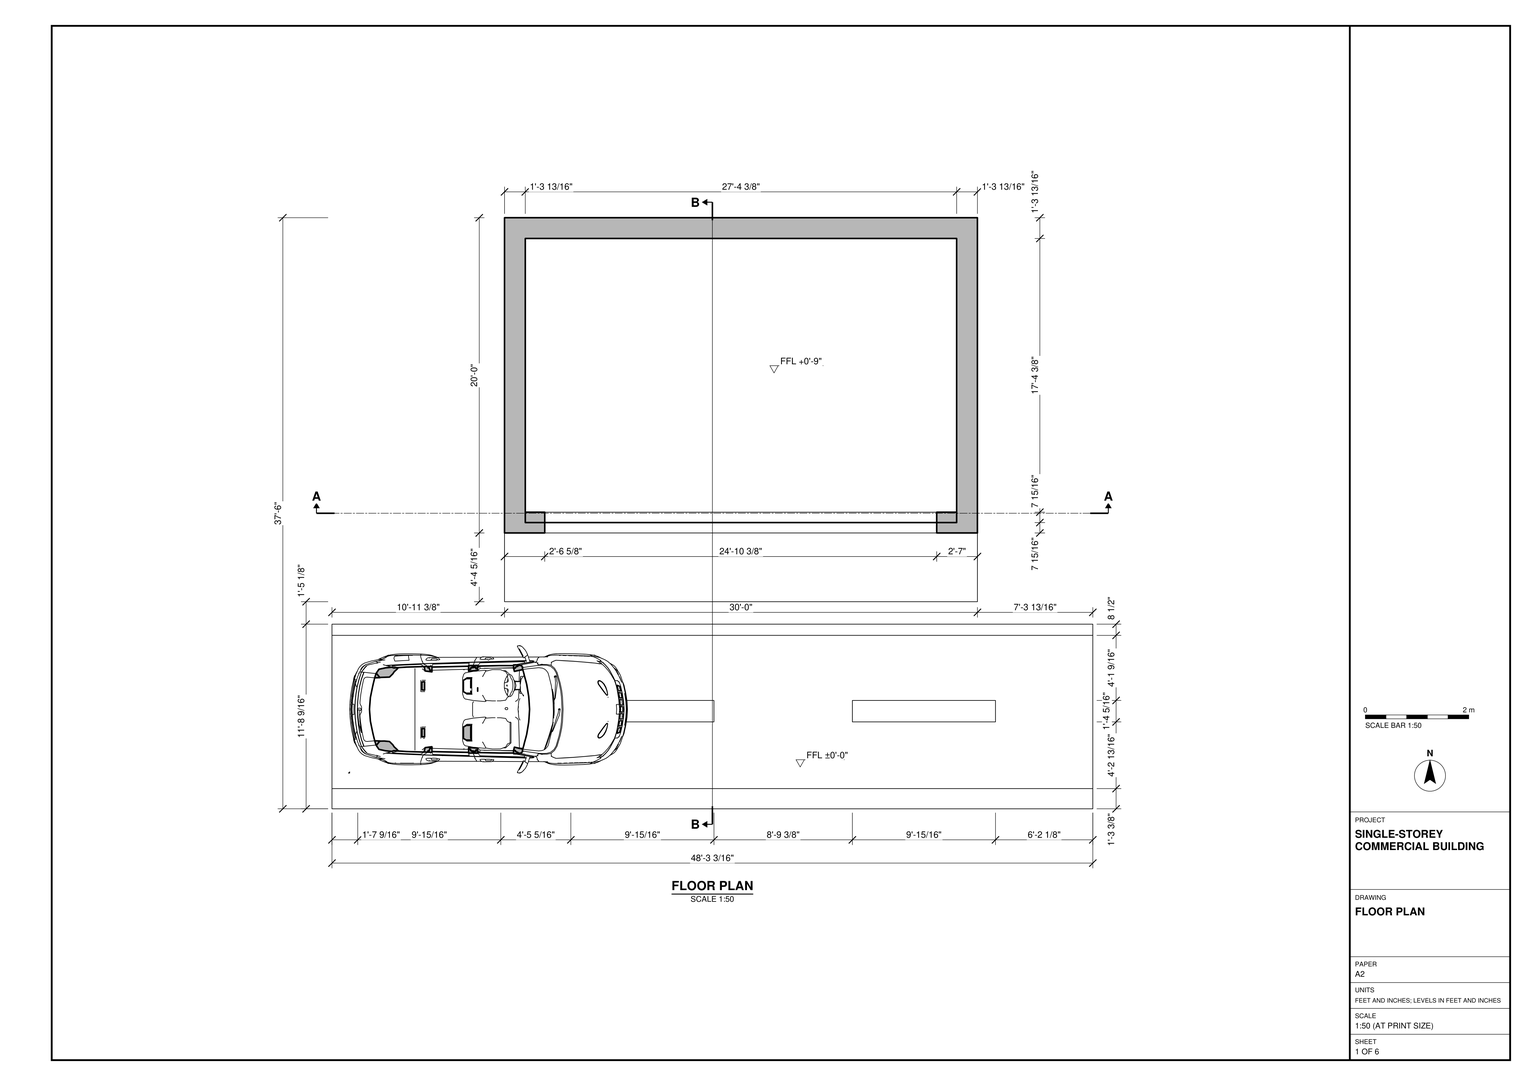
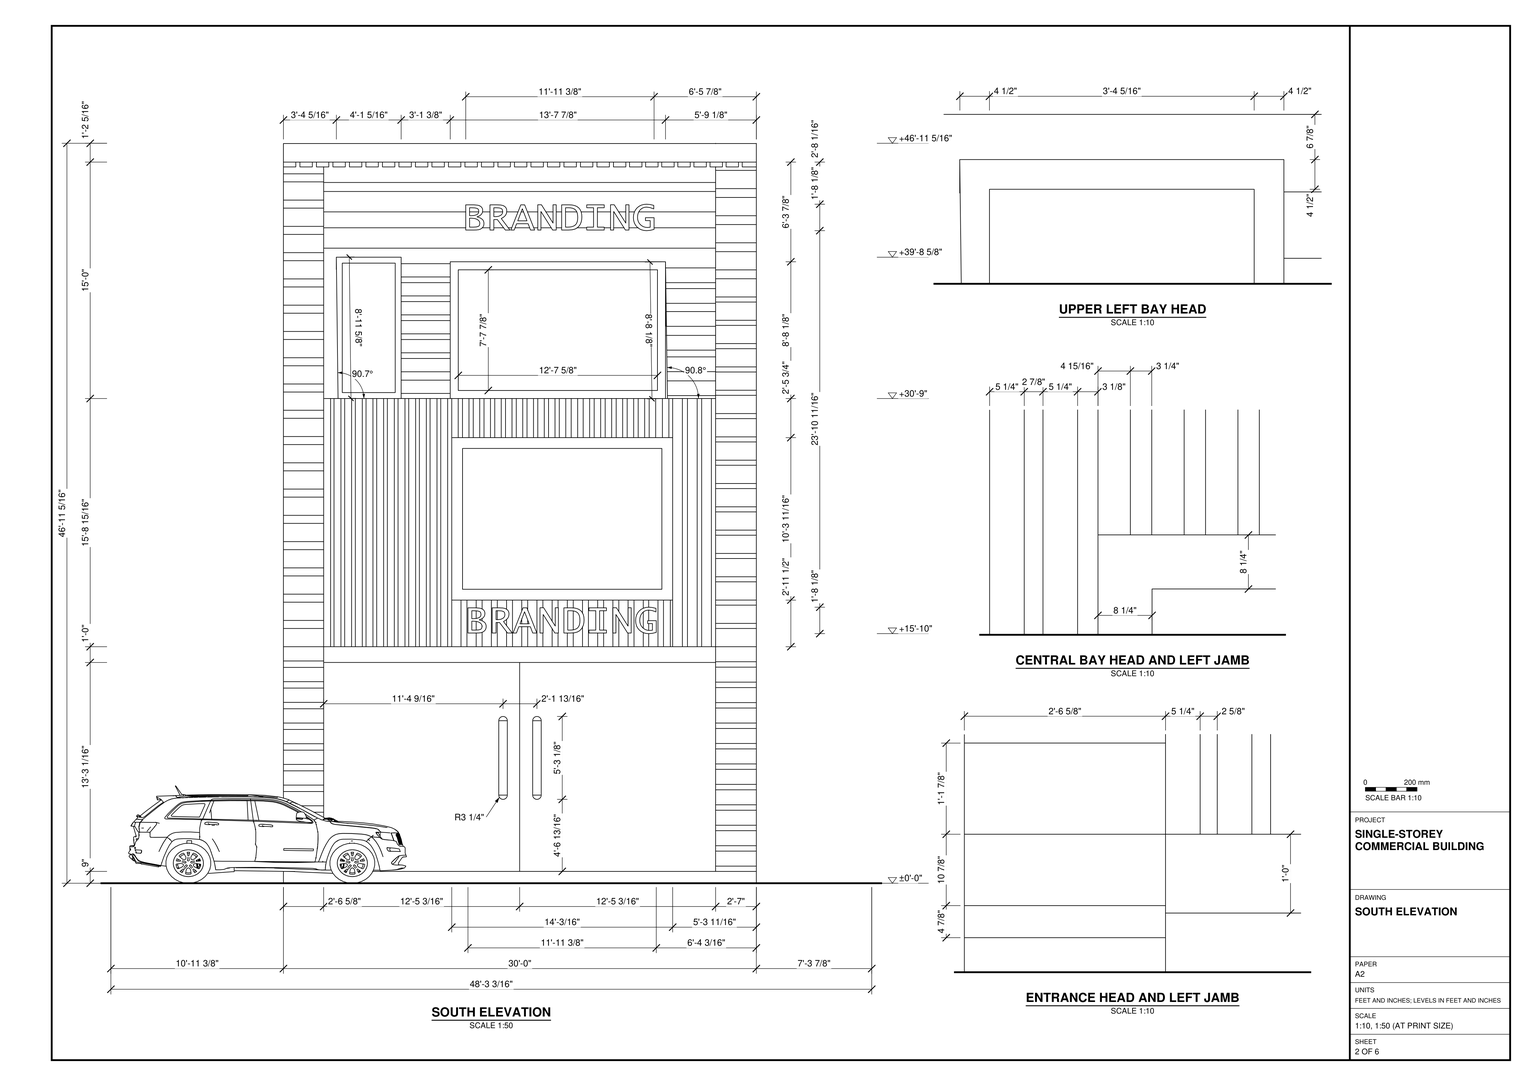
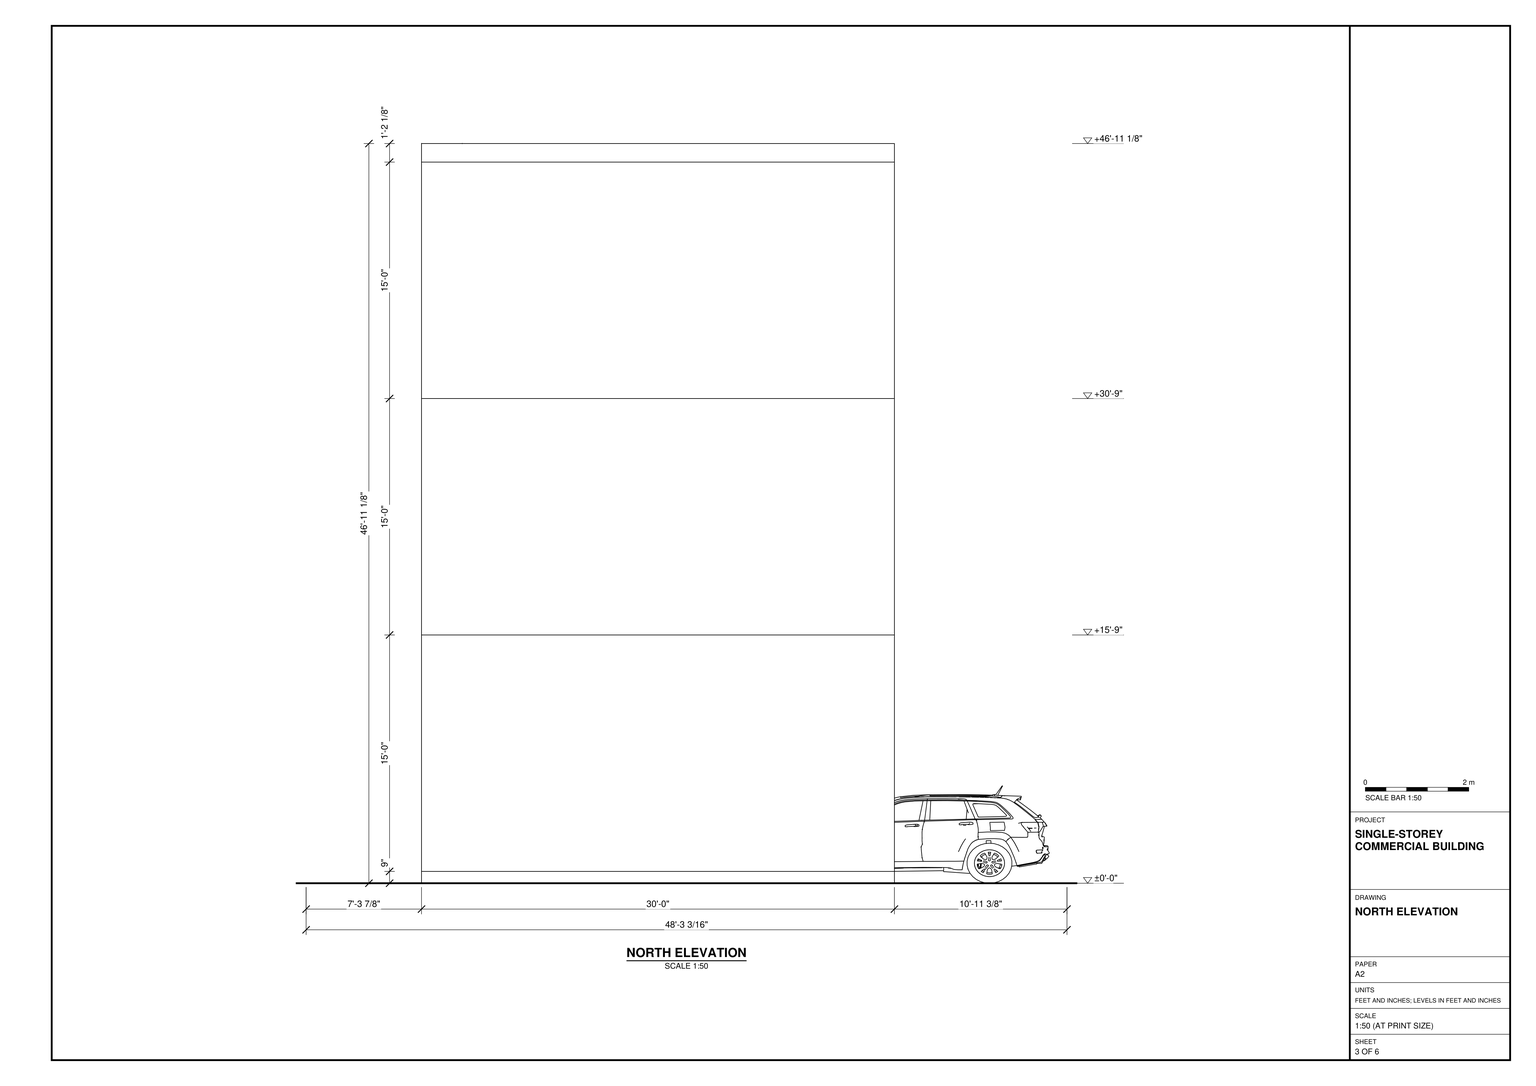
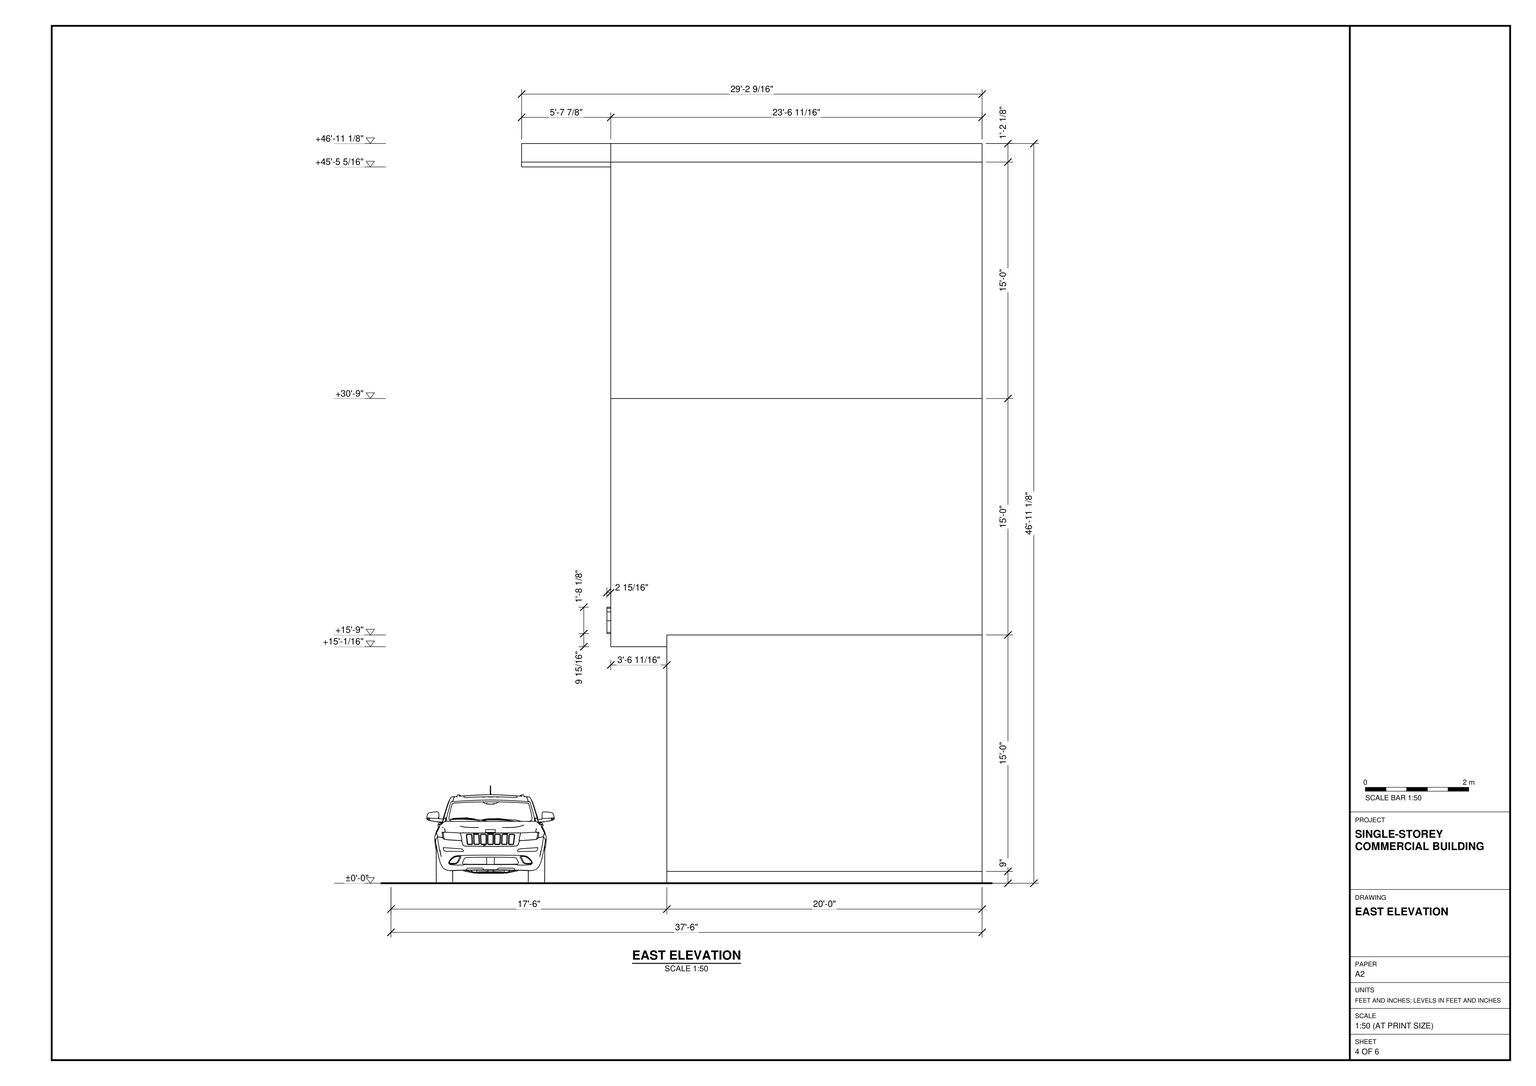
Use task_files/diagram_01.pdf to model the building and its forecourt in SketchUp. Work in feet and inches. The complete model measures 48'-3 3/16" along x, 37'-6" along y and 46'-11 1/8" along z. Use ±0'-0" as the ground datum at the forecourt. Set the building's finished floor at +0'-9". Keep the building single-storey: the horizontal divisions on the elevations are not additional storeys.

Set out the 30'-0" by 20'-0" rectangular shell behind the forecourt, using the setbacks and wall thicknesses on the floor plan. Model the raised floor slab, walls and flat roof with its cap. On the south face, frame the wide entrance between the banded side piers and place a vertical pull on each door leaf. Above the entrance, model the vertically ribbed field around the central framed bay. Use horizontal courses around the upper bays, with the narrow bay on the left and the wider bay to its right. Follow the enlarged details for the heads and jambs, and place the sign lettering as shown. Keep the rear face plain apart from its horizontal divisions.

Include the forecourt markings and the car near the left end in plan. Decor and loose items, including the car, may be any suitable library components. Keep walls, slabs, roof and each joinery or furniture piece in separate groups or components, and use components for repeated parts. Save one SketchUp model as output_files/single_storey_commercial_building_with_storefront.skp.

# SketchUp Ruby script. Lengths in inches.
U = 1.inch
M = Sketchup.active_model
def pt(a) = Geom::Point3d.new(a.map { |v| v * U })
def face(e, loops, mat)
  f = e.add_face(loops[0].map { |a| pt(a) })
  loops[1..].each { |l| e.add_face(l.map { |a| pt(a) }).erase! }
  f.material = f.back_material = mat if mat
  f
end
# faces: each face lists its corners as indices into pts; further lists are holes
def faces(e, pts, list, mat = nil) = list.each { |f| face(e, (f[0].is_a?(Array) ? f : [f]).map { |l| l.map { |i| pts[i] } }, mat) }
# xy, xz, yz: faces in a plane at the given z, y or x. An outline is a flat list of corners, or four numbers for a rectangle; further outlines are holes
def ring(l) = l.size == 4 ? [[l[0], l[1]], [l[2], l[1]], [l[2], l[3]], [l[0], l[3]]] : l.each_slice(2).to_a
def flat(e, list, mat, &to3) = list.each { |f| face(e, (f[0].is_a?(Array) ? f : [f]).map { |l| ring(l).map { |u, v| to3.(u, v) } }, mat) }
def xy(e, z, list, mat = nil) = flat(e, list, mat) { |x, y| [x, y, z] }
def xz(e, y, list, mat = nil) = flat(e, list, mat) { |x, z| [x, y, z] }
def yz(e, x, list, mat = nil) = flat(e, list, mat) { |y, z| [x, y, z] }
def lines(e, pts, list) = list.each { |a, b| e.add_line(pt(pts[a]), pt(pts[b])) }
# prism: a flat outline (further loops are holes) pulled along v
def prism(e, loops, v, mat = nil)
  f = face(e, loops, mat); d = Geom::Vector3d.new(v.map { |x| x * U })
  f.pushpull(f.normal.samedirection?(d) ? d.length : -d.length)
end
def box(e, o, s, mat = nil) = prism(e, [[o, [o[0] + s[0], o[1], o[2]], [o[0] + s[0], o[1] + s[1], o[2]], [o[0], o[1] + s[1], o[2]]]], [0, 0, s[2]], mat)
def at(x, y, z, deg = 0) = Geom::Transformation.translation(pt([x, y, z])) * Geom::Transformation.rotation(ORIGIN, Z_AXIS, deg.degrees)
def axes(o, x, y, z) = Geom::Transformation.new([*x, 0, *y, 0, *z, 0, *pt(o).to_a, 1])
def part(name) = M.definitions.add(name)
# library, detail: a bought-in or finely detailed component or shape, given as its bounding box
def library(name, o, s) = part(name).tap { |d| box(d.entities, o, s) }
def detail(e, o, s) = box(e.add_group.entities, o, s)
def put(e, d, t, mat = nil) = e.add_instance(d, t).tap { |i| i.material = mat if mat }
def group(e, t, mat = nil) = e.add_group.tap { |g| g.transformation = t; g.material = mat if mat }.entities
root = M.entities
M.materials.add("[Color M00]").color = [255, 255, 255]
M.materials.add("[Color M06]").color = [86, 86, 86]
M.materials.add("[Formica Beige]").color = [211, 187, 149]
M.materials.add("[Formica Laminate Dark]").color = [50, 53, 60]
M.materials.add("[Formica Speckled Grey]").color = [94, 105, 111]
M.materials.add("[Herringbone 4x1]").color = [216, 216, 216]
M.materials.add("[Quartz Light Brown]").color = [199, 184, 152]
M.materials.add("[Quartz Light Grey]").color = [251, 251, 252]
M.materials.add("[Terrazzo Light Blue]").color = [196, 214, 227]
M.materials.add("[Terrazzo Tile Light]").color = [219, 217, 210]
M.materials.add("[Translucent Glass Gray]").color = [128, 128, 128]
M.materials["[Translucent Glass Gray]"].alpha = 0.5
M.materials.add("[Translucent Glass Safety]").color = [204, 235, 244]
M.materials["[Translucent Glass Safety]"].alpha = 0.5
M.materials.add("[Translucent Glass Sky Reflection]").color = [126, 138, 183]
M.materials["[Translucent Glass Sky Reflection]"].alpha = 0.52
M.materials.add("[Wood Cherry Original]").color = [112, 63, 31]
M.materials.add("[Wood Cherry Original]1").color = [112, 63, 31]
M.materials.add("[Wood Veneer 01]").color = [56, 32, 17]
M.materials.add("[Wood Veneer 01]1").color = [43, 25, 13]
c1 = library("skpE847",[-111.76,-15.01,0.76],[2.12,4.6,1.82])
c2 = part("car+1")
p = [[0,0,0],[1,0,0],[1,1,0]]
lines(c2.entities,p,[[0,1],[1,2],[2,0]])
put(c2.entities,c1,axes([-477.97,5140.8,-31.25],[0,46,0],[-46,0,0],[0,0,40.94]))
c3 = library("BRANDING",[2.77,0,0],[143.37,20.125,12])
c4 = library("BRANDING\#1",[2.77,0,0],[143.37,20.125,12])
xy(root,0,[[0,0,579.1875,15.375],[0,132.05,579.1875,140.5625],[131.35,210,491.35,450]])
xy(root,0,[[19.59,66.17,128.53,82.48],[181.84,66.17,290.78,82.48],[396.15,66.17,505.09,82.48]],"[Color M00]")
xy(root,0,[[[0,15.375,579.1875,132.05],[19.59,66.17,128.53,82.48],[181.84,66.17,290.78,82.48],[396.15,66.17,505.09,82.48]]],"[Color M06]")
xy(root,0,[[131.35,157.67,491.35,210]],"[Terrazzo Tile Light]")
xy(root,9,[[131.35,210,131.35,450,491.35,450,491.35,210,460.35,210,460.35,217.91,475.53,217.91,475.53,434.1875,147.16,434.1875,147.16,217.91,161.98,217.91,161.98,210],[161.98,210,460.35,217.91],[147.16,217.91,161.98,225.82],[161.98,217.91,460.35,225.82],[460.35,217.91,475.53,225.82],
  [147.16,225.82,475.53,434.1875]])
xy(root,168.0625,[[161.98,217.91,460.35,225.82]])
xy(root,180.0625,[[161.98,169.07,167.25,172.19],[169.85,169.07,175.12,172.19],[177.98,169.07,183.25,172.19],[186.1,169.07,191.37,172.19],[194.23,169.07,199.5,172.19],
  [202.35,169.07,207.62,172.19],[210.48,169.07,215.75,172.19],[218.6,169.07,223.87,172.19],[226.73,169.07,232,172.19],[234.85,169.07,240.12,172.19],
  [242.98,169.07,248.25,172.19],[251.1,169.07,256.37,172.19],[259.48,169.07,266.52,172.19],[271.04,169.07,278.08,172.19],[282.6,169.07,289.65,172.19],
  [294.16,169.07,301.21,172.19],[305.73,169.07,312.77,172.19],[317.29,169.07,324.33,172.19],[328.85,169.07,335.9,172.19],[340.41,169.07,347.46,172.19],
  [351.98,169.07,359.02,172.19],[363.54,169.07,370.58,172.19],[375.1,169.07,382.15,172.19],[386.66,169.07,393.71,172.19],[398.23,169.07,405.27,172.19],
  [409.42,169.07,416.47,172.19],[420.67,169.07,425.87,172.19],[427.66,169.07,435.06,172.19],[438.91,169.07,446.31,172.19],[449.73,169.07,457.12,172.19],
  [147.16,210,161.98,217.91],[460.35,210,475.53,217.91]])
xy(root,180.0625,[[131.35,167.32,131.35,210,147.16,210,147.16,172.19,161.98,172.19,161.98,167.32],[460.35,167.32,460.35,172.19,475.53,172.19,475.53,210,491.35,210,491.35,167.32],[147.16,172.19,147.16,210,161.98,210,161.98,217.91,460.35,217.91,460.35,210,475.53,210,475.53,172.19]],"[Terrazzo Light Blue]")
xy(root,189,[[131.35,210,131.35,450,491.35,450,491.35,210,475.53,210,475.53,434.1875,147.16,434.1875,147.16,210],[147.16,217.91,161.98,225.82],[161.98,217.91,460.35,225.82],[460.35,217.91,475.53,225.82],[147.16,225.82,475.53,434.1875]])
xy(root,215.54,[[259.48,172.19,427.66,184.32]])
xy(root,215.54,[[259.48,169.07,266.52,172.19],[271.04,169.07,278.08,172.19],[282.6,169.07,289.65,172.19],[294.16,169.07,301.21,172.19],[305.73,169.07,312.77,172.19],
  [317.29,169.07,324.33,172.19],[328.85,169.07,335.9,172.19],[340.41,169.07,347.46,172.19],[351.98,169.07,359.02,172.19],[363.54,169.07,370.58,172.19],
  [375.1,169.07,382.15,172.19],[386.66,169.07,393.71,172.19],[398.23,169.07,405.27,172.19],[409.42,169.07,416.47,172.19],[420.67,169.07,425.87,172.19]],"[Formica Laminate Dark]")
xy(root,339.23,[[259.48,169.07,264.41,172.19],[267.66,169.07,272.59,172.19],[275.85,169.07,280.78,172.19],[284.04,169.07,288.97,172.19],[292.23,169.07,297.16,172.19],
  [300.41,169.07,305.34,172.19],[308.6,169.07,313.53,172.19],[316.79,169.07,321.72,172.19],[324.98,169.07,329.91,172.19],[333.16,169.07,338.09,172.19],
  [341.35,169.07,346.28,172.19],[350.41,169.07,355.34,172.19],[359.54,169.07,364.47,172.19],[367.91,169.07,372.84,172.19],[376.29,169.07,381.22,172.19],
  [384.66,169.07,389.59,172.19],[393.04,169.07,397.97,172.19],[401.41,169.07,406.34,172.19],[409.79,169.07,414.72,172.19],[419.85,169.07,424.78,172.19],
  [259.48,172.19,427.66,184.32]])
xy(root,369,[[147.16,172.19,147.16,434.1875,475.53,434.1875,475.53,172.19,423.7,172.19,422.2,183.13,258.32,183.13,258.32,172.19,220.97,172.19,220.97,178.82,171.61,178.82,172.93,172.19]])
xy(root,369,[[161.98,169.07,167.25,172.19],[169.85,169.07,172.93,172.19],[172.93,169.07,175.12,172.19],[177.98,169.07,181.05,172.19],[181.05,169.07,183.25,172.19],
  [186.1,169.07,189.18,172.19],[189.18,169.07,191.37,172.19],[194.23,169.07,197.3,172.19],[197.3,169.07,199.5,172.19],[202.35,169.07,205.43,172.19],
  [205.43,169.07,207.62,172.19],[210.48,169.07,213.55,172.19],[213.55,169.07,215.75,172.19],[218.6,169.07,220.97,172.19],[220.97,169.07,221.68,172.19],
  [221.68,169.07,223.87,172.19],[226.73,169.07,229.8,172.19],[229.8,169.07,232,172.19],[234.85,169.07,237.93,172.19],[237.93,169.07,240.12,172.19],
  [242.98,169.07,246.05,172.19],[246.05,169.07,248.25,172.19],[251.1,169.07,254.18,172.19],[254.18,169.07,256.37,172.19],[259.48,169.07,264.41,172.19],
  [267.66,169.07,272.59,172.19],[275.85,169.07,280.78,172.19],[284.04,169.07,288.97,172.19],[292.23,169.07,297.16,172.19],[300.41,169.07,305.34,172.19],
  [308.6,169.07,313.53,172.19],[316.79,169.07,321.72,172.19],[324.98,169.07,329.91,172.19],[333.16,169.07,338.09,172.19],[341.35,169.07,346.28,172.19],
  [350.41,169.07,355.34,172.19],[359.54,169.07,364.47,172.19],[367.91,169.07,372.84,172.19],[376.29,169.07,381.22,172.19],[384.66,169.07,389.59,172.19],
  [393.04,169.07,397.97,172.19],[401.41,169.07,406.34,172.19],[409.79,169.07,414.72,172.19],[419.85,169.07,423.7,172.19],[423.7,169.07,424.78,172.19],
  [427.66,169.07,435.06,172.19],[438.91,169.07,446.31,172.19],[449.73,169.07,457.12,172.19]],"[Formica Laminate Dark]")
xy(root,369,[[172.93,172.19,171.61,178.82,220.97,178.82,220.97,172.19],[258.32,172.19,258.32,183.13,422.2,183.13,423.7,172.19]],"[Quartz Light Grey]")
xy(root,473.125,[[258.32,172.19,422.2,183.13]])
xy(root,476.6,[[171.61,172.19,220.97,178.82]])
xy(root,545.3125,[[131.35,99.44,140.77,167.32],[143.91,99.44,153.33,167.32],[156.47,99.44,165.9,167.32],[169.03,99.44,178.46,167.32],[181.6,99.44,191.02,167.32],
  [194.16,99.44,203.58,167.32],[206.72,99.44,216.15,167.32],[219.28,99.44,228.71,167.32],[231.85,99.44,241.27,167.32],[244.41,99.44,253.83,167.32],
  [256.97,99.44,266.4,167.32],[269.53,99.44,278.96,167.32],[282.1,99.44,291.52,167.32],[294.66,99.44,304.08,167.32],[307.22,99.44,316.65,167.32],
  [319.78,99.44,329.21,167.32],[332.35,99.44,341.77,167.32],[344.91,99.44,354.33,167.32],[357.47,99.44,366.9,167.32],[370.03,99.44,379.46,167.32],
  [382.6,99.44,392.02,167.32],[394.85,99.44,404.27,167.32],[407.1,99.44,416.52,167.32],[419.35,99.44,428.77,167.32],[431.6,99.44,441.02,167.32],
  [443.85,99.44,453.27,167.32],[456.1,99.44,465.52,167.32],[468.35,99.44,477.77,167.32],[480.6,99.44,491.35,167.32]],"[Wood Veneer 01]")
xy(root,549,[[131.35,99.44,140.77,167.32],[140.77,99.44,143.91,167.32],[143.91,99.44,153.33,167.32],[153.33,99.44,156.47,167.32],[156.47,99.44,165.9,167.32],
  [165.9,99.44,169.03,167.32],[169.03,99.44,178.46,167.32],[178.46,99.44,181.6,167.32],[181.6,99.44,191.02,167.32],[191.02,99.44,194.16,167.32],
  [194.16,99.44,203.58,167.32],[203.58,99.44,206.72,167.32],[206.72,99.44,216.15,167.32],[216.15,99.44,219.28,167.32],[219.28,99.44,228.71,167.32],
  [228.71,99.44,231.85,167.32],[231.85,99.44,241.27,167.32],[241.27,99.44,244.41,167.32],[244.41,99.44,253.83,167.32],[253.83,99.44,256.97,167.32],
  [256.97,99.44,266.4,167.32],[266.4,99.44,269.53,167.32],[269.53,99.44,278.96,167.32],[278.96,99.44,282.1,167.32],[282.1,99.44,291.52,167.32],
  [291.52,99.44,294.66,167.32],[294.66,99.44,304.08,167.32],[304.08,99.44,307.22,167.32],[307.22,99.44,316.65,167.32],[316.65,99.44,319.78,167.32],
  [319.78,99.44,329.21,167.32],[329.21,99.44,332.35,167.32],[332.35,99.44,341.77,167.32],[341.77,99.44,344.91,167.32],[344.91,99.44,354.33,167.32],
  [354.33,99.44,357.47,167.32],[357.47,99.44,366.9,167.32],[366.9,99.44,370.03,167.32],[370.03,99.44,379.46,167.32],[379.46,99.44,382.6,167.32],
  [382.6,99.44,392.02,167.32],[392.02,99.44,394.85,167.32],[394.85,99.44,404.27,167.32],[404.27,99.44,407.1,167.32],[407.1,99.44,416.52,167.32],
  [416.52,99.44,419.35,167.32],[419.35,99.44,428.77,167.32],[428.77,99.44,431.6,167.32],[431.6,99.44,441.02,167.32],[441.02,99.44,443.85,167.32],
  [443.85,99.44,453.27,167.32],[453.27,99.44,456.1,167.32],[456.1,99.44,465.52,167.32],[465.52,99.44,468.35,167.32],[468.35,99.44,477.77,167.32],
  [477.77,99.44,480.6,167.32],[480.6,99.44,491.35,167.32],[131.35,167.32,147.16,450],[147.16,167.32,161.98,172.19],[161.98,167.32,460.35,172.19],
  [460.35,167.32,475.53,172.19],[475.53,167.32,491.35,450],[147.16,172.19,475.53,434.1875],[147.16,434.1875,475.53,450]])
xy(root,563.125,[[131.35,99.44,491.35,450]],"[Wood Veneer 01]1")
xz(root,99.44,[[131.35,545.3125,140.77,549],[143.91,545.3125,153.33,549],[156.47,545.3125,165.9,549],[169.03,545.3125,178.46,549],[181.6,545.3125,191.02,549],
  [194.16,545.3125,203.58,549],[206.72,545.3125,216.15,549],[219.28,545.3125,228.71,549],[231.85,545.3125,241.27,549],[244.41,545.3125,253.83,549],
  [256.97,545.3125,266.4,549],[269.53,545.3125,278.96,549],[282.1,545.3125,291.52,549],[294.66,545.3125,304.08,549],[307.22,545.3125,316.65,549],
  [319.78,545.3125,329.21,549],[332.35,545.3125,341.77,549],[344.91,545.3125,354.33,549],[357.47,545.3125,366.9,549],[370.03,545.3125,379.46,549],
  [382.6,545.3125,392.02,549],[394.85,545.3125,404.27,549],[407.1,545.3125,416.52,549],[419.35,545.3125,428.77,549],[431.6,545.3125,441.02,549],
  [443.85,545.3125,453.27,549],[456.1,545.3125,465.52,549],[468.35,545.3125,477.77,549],[480.6,545.3125,491.35,549]],"[Wood Veneer 01]")
xz(root,99.44,[[131.35,549,491.35,563.125]],"[Wood Veneer 01]1")
xz(root,167.32,[[131.35,545.3125,140.77,549],[143.91,545.3125,147.16,549],[143.91,545.3125,153.33,549],[147.16,545.3125,153.33,549],[156.47,545.3125,161.98,549],
  [161.98,545.3125,165.9,549],[169.03,545.3125,178.46,549],[181.6,545.3125,191.02,549],[194.16,545.3125,203.58,549],[206.72,545.3125,216.15,549],
  [219.28,545.3125,228.71,549],[231.85,545.3125,241.27,549],[244.41,545.3125,253.83,549],[256.97,545.3125,266.4,549],[269.53,545.3125,278.96,549],
  [282.1,545.3125,291.52,549],[294.66,545.3125,304.08,549],[307.22,545.3125,316.65,549],[319.78,545.3125,329.21,549],[332.35,545.3125,341.77,549],
  [344.91,545.3125,354.33,549],[357.47,545.3125,366.9,549],[370.03,545.3125,379.46,549],[382.6,545.3125,392.02,549],[394.85,545.3125,404.27,549],
  [407.1,545.3125,416.52,549],[419.35,545.3125,428.77,549],[431.6,545.3125,441.02,549],[443.85,545.3125,453.27,549],[456.1,545.3125,460.35,549],
  [460.35,545.3125,465.52,549],[468.35,545.3125,475.53,549],[475.53,545.3125,477.77,549],[480.6,545.3125,491.35,549],[131.35,549,161.98,553.95]])
xz(root,167.32,[[131.35,193.95,161.98,200.0625],[460.35,193.95,491.35,197.8125],[460.35,211.7,491.35,215.5625],[131.35,213.95,161.98,220.0625],[460.35,229.45,491.35,233.3125],
  [131.35,233.95,161.98,240.0625],[460.35,247.2,491.35,251.0625],[131.35,253.95,161.98,260.0625],[460.35,264.95,491.35,268.8125],[131.35,273.95,161.98,280.0625],
  [460.35,282.7,491.35,286.5625],[131.35,293.95,161.98,300.0625],[460.35,300.45,491.35,304.3125],[131.35,313.95,161.98,320.0625],[460.35,318.2,491.35,322.0625],
  [131.35,333.95,161.98,340.0625],[460.35,335.95,491.35,339.8125],[460.35,353.7,491.35,357.5625],[131.35,353.95,161.98,360.0625],[460.35,371.45,491.35,375.3125],
  [131.35,373.95,161.98,380.0625],[460.35,389.2,491.35,393.0625],[131.35,393.95,161.98,400.0625],[460.35,406.95,491.35,410.8125],[131.35,413.95,161.98,420.0625],
  [460.35,424.7,491.35,428.5625],[131.35,433.95,161.98,440.0625],[460.35,442.45,491.35,446.3125],[131.35,453.95,161.98,460.0625],[460.35,460.2,491.35,466.9375],
  [131.35,473.95,161.98,480.0625],[460.35,480.82,491.35,487.5625],[131.35,493.95,161.98,500.0625],[460.35,501.45,491.35,508.1875],[131.35,513.95,161.98,520.0625],
  [460.35,522.07,491.35,528.8125],[131.35,533.95,161.98,540.0625],[460.35,542.7,491.35,542.7,491.35,545.3125,480.6,545.3125,480.6,549,477.77,549,477.77,545.3125,468.35,545.3125,468.35,549,465.52,549,465.52,545.3125,460.35,545.3125]],"[Formica Laminate Dark]")
xz(root,167.32,[[131.35,180.0625,161.98,193.95],[460.35,180.0625,491.35,193.95],[460.35,197.8125,491.35,211.7],[131.35,200.0625,161.98,213.95],[460.35,215.5625,491.35,229.45],
  [131.35,220.0625,161.98,233.95],[460.35,233.3125,491.35,247.2],[131.35,240.0625,161.98,253.95],[460.35,251.0625,491.35,264.95],[131.35,260.0625,161.98,273.95],
  [460.35,268.8125,491.35,282.7],[131.35,280.0625,161.98,293.95],[460.35,286.5625,491.35,300.45],[131.35,300.0625,161.98,313.95],[460.35,304.3125,491.35,318.2],
  [131.35,320.0625,161.98,333.95],[460.35,322.0625,491.35,335.95],[460.35,339.8125,491.35,353.7],[131.35,340.0625,161.98,353.95],[460.35,357.5625,491.35,371.45],
  [131.35,360.0625,161.98,373.95],[460.35,375.3125,491.35,389.2],[131.35,380.0625,161.98,393.95],[460.35,393.0625,491.35,406.95],[131.35,400.0625,161.98,413.95],
  [460.35,410.8125,491.35,424.7],[131.35,420.0625,161.98,433.95],[460.35,428.5625,491.35,442.45],[131.35,440.0625,161.98,453.95],[460.35,446.3125,491.35,460.2],
  [131.35,460.0625,161.98,473.95],[460.35,466.9375,491.35,480.82],[131.35,480.0625,161.98,493.95],[460.35,487.5625,491.35,501.45],[131.35,500.0625,161.98,513.95],
  [460.35,508.1875,491.35,522.07],[131.35,520.0625,161.98,533.95],[460.35,528.8125,491.35,542.7],[131.35,540.0625,161.98,540.0625,161.98,545.3125,156.47,545.3125,156.47,549,153.33,549,153.33,545.3125,143.91,545.3125,143.91,549,140.77,549,140.77,545.3125,131.35,545.3125]],"[Wood Cherry Original]")
xz(root,169.07,[[161.98,180.0625,167.25,369],[169.85,180.0625,175.12,369],[177.98,180.0625,183.25,369],[186.1,180.0625,191.37,369],[194.23,180.0625,199.5,369],
  [202.35,180.0625,207.62,369],[210.48,180.0625,215.75,369],[218.6,180.0625,223.87,369],[226.73,180.0625,232,369],[234.85,180.0625,240.12,369],
  [242.98,180.0625,248.25,369],[251.1,180.0625,256.37,369],[259.48,180.0625,266.52,215.54],[271.04,180.0625,278.08,215.54],[282.6,180.0625,289.65,215.54],
  [294.16,180.0625,301.21,215.54],[305.73,180.0625,312.77,215.54],[317.29,180.0625,324.33,215.54],[328.85,180.0625,335.9,215.54],[340.41,180.0625,347.46,215.54],
  [351.98,180.0625,359.02,215.54],[363.54,180.0625,370.58,215.54],[375.1,180.0625,382.15,215.54],[386.66,180.0625,393.71,215.54],[398.23,180.0625,405.27,215.54],
  [409.42,180.0625,416.47,215.54],[420.67,180.0625,425.87,215.54],[427.66,180.0625,435.06,369],[438.91,180.0625,446.31,369],[449.73,180.0625,457.12,369],
  [259.48,339.23,264.41,369],[267.66,339.23,272.59,369],[275.85,339.23,280.78,369],[284.04,339.23,288.97,369],[292.23,339.23,297.16,369],
  [300.41,339.23,305.34,369],[308.6,339.23,313.53,369],[316.79,339.23,321.72,369],[324.98,339.23,329.91,369],[333.16,339.23,338.09,369],
  [341.35,339.23,346.28,369],[350.41,339.23,355.34,369],[359.54,339.23,364.47,369],[367.91,339.23,372.84,369],[376.29,339.23,381.22,369],
  [384.66,339.23,389.59,369],[393.04,339.23,397.97,369],[401.41,339.23,406.34,369],[409.79,339.23,414.72,369],[419.85,339.23,424.78,369]],"[Formica Laminate Dark]")
xz(root,172.19,[[147.16,180.0625,161.98,369],[161.98,180.0625,167.25,369],[169.85,180.0625,175.12,369],[177.98,180.0625,183.25,369],[186.1,180.0625,191.37,369],
  [194.23,180.0625,199.5,369],[202.35,180.0625,207.62,369],[210.48,180.0625,215.75,369],[218.6,180.0625,223.87,369],[226.73,180.0625,232,369],
  [234.85,180.0625,240.12,369],[242.98,180.0625,248.25,369],[251.1,180.0625,256.37,369],[259.48,180.0625,266.52,215.54],[271.04,180.0625,278.08,215.54],
  [282.6,180.0625,289.65,215.54],[294.16,180.0625,301.21,215.54],[305.73,180.0625,312.77,215.54],[317.29,180.0625,324.33,215.54],[328.85,180.0625,335.9,215.54],
  [340.41,180.0625,347.46,215.54],[351.98,180.0625,359.02,215.54],[363.54,180.0625,370.58,215.54],[375.1,180.0625,382.15,215.54],[386.66,180.0625,393.71,215.54],
  [398.23,180.0625,405.27,215.54],[409.42,180.0625,416.47,215.54],[420.67,180.0625,425.87,215.54],[427.66,180.0625,435.06,369],[438.91,180.0625,446.31,369],
  [449.73,180.0625,457.12,369],[460.35,180.0625,475.53,369],[259.48,339.23,264.41,369],[267.66,339.23,272.59,369],[275.85,339.23,280.78,369],
  [284.04,339.23,288.97,369],[292.23,339.23,297.16,369],[300.41,339.23,305.34,369],[308.6,339.23,313.53,369],[316.79,339.23,321.72,369],
  [324.98,339.23,329.91,369],[333.16,339.23,338.09,369],[341.35,339.23,346.28,369],[350.41,339.23,355.34,369],[359.54,339.23,364.47,369],
  [367.91,339.23,372.84,369],[376.29,339.23,381.22,369],[384.66,339.23,389.59,369],[393.04,339.23,397.97,369],[401.41,339.23,406.34,369],
  [409.79,339.23,414.72,369],[419.85,339.23,424.78,369],[147.16,369,161.98,549],[460.35,369,475.53,549],[422.66,423.96,422.91,423.96,422.75,435.2,422.49,435.2]])
xz(root,172.19,[[423.51,382.45,460.35,382.45,460.35,389.46,423.4,389.46],[220.97,382.98,258.32,389.37],[220.97,399.48,258.32,403.81],[423.24,400.7,460.35,400.7,460.35,405.84,423.17,405.84],[220.97,413.92,258.32,418.25],
  [423.01,417.07,460.35,417.07,460.35,423.96,422.91,423.96],[220.97,428.36,258.32,432.68],[422.75,435.2,460.35,435.2,460.35,441.46,422.66,441.46],[220.97,442.79,258.32,447.12],[422.49,452.7,460.35,452.7,460.35,457.21,422.43,457.21],
  [220.97,457.23,258.32,461.56],[161.98,499,460.35,511.1],[161.98,526.625,460.35,533.48]],"[Formica Laminate Dark]")
xz(root,172.19,[[167.25,180.0625,169.85,369],[175.12,180.0625,177.98,369],[183.25,180.0625,186.1,369],[191.37,180.0625,194.23,369],[199.5,180.0625,202.35,369],
  [207.62,180.0625,210.48,369],[215.75,180.0625,218.6,369],[223.87,180.0625,226.73,369],[232,180.0625,234.85,369],[240.12,180.0625,242.98,369],
  [248.25,180.0625,251.1,369],[256.37,180.0625,259.48,369],[266.52,180.0625,271.04,215.54],[278.08,180.0625,282.6,215.54],[289.65,180.0625,294.16,215.54],
  [301.21,180.0625,305.73,215.54],[312.77,180.0625,317.29,215.54],[324.33,180.0625,328.85,215.54],[335.9,180.0625,340.41,215.54],[347.46,180.0625,351.98,215.54],
  [359.02,180.0625,363.54,215.54],[370.58,180.0625,375.1,215.54],[382.15,180.0625,386.66,215.54],[393.71,180.0625,398.23,215.54],[405.27,180.0625,409.42,215.54],
  [416.47,180.0625,420.67,215.54],[425.87,180.0625,427.66,215.54],[435.06,180.0625,438.91,369],[446.31,180.0625,449.73,369],[457.12,180.0625,460.35,369],
  [264.41,339.23,267.66,369],[272.59,339.23,275.85,369],[280.78,339.23,284.04,369],[288.97,339.23,292.23,369],[297.16,339.23,300.41,369],
  [305.34,339.23,308.6,369],[313.53,339.23,316.79,369],[321.72,339.23,324.98,369],[329.91,339.23,333.16,369],[338.09,339.23,341.35,369],
  [346.28,339.23,350.41,369],[355.34,339.23,359.54,369],[364.47,339.23,367.91,369],[372.84,339.23,376.29,369],[381.22,339.23,384.66,369],
  [389.59,339.23,393.04,369],[397.97,339.23,401.41,369],[406.34,339.23,409.79,369],[414.72,339.23,419.85,369],[424.78,339.23,427.66,369],
  [220.97,369,258.32,372.87],[423.7,369,460.35,369,460.35,371.21,423.67,371.21]],"[Formica Speckled Grey]")
xz(root,172.19,[[161.98,369,172.93,369,171.61,476.6,220.97,476.6,220.97,471.67,258.32,471.67,258.32,473.125,422.2,473.125,422.27,468.45,460.35,468.45,460.35,483.48,161.98,483.48],[423.67,371.21,460.35,371.21,460.35,382.45,423.51,382.45],[220.97,372.87,258.32,382.98],[220.97,389.37,258.32,399.48],[423.4,389.46,460.35,389.46,460.35,400.7,423.24,400.7],
  [220.97,403.81,258.32,413.92],[423.17,405.84,460.35,405.84,460.35,417.07,423.01,417.07],[220.97,418.25,258.32,428.36],[422.91,423.96,460.35,423.96,460.35,435.2,422.75,435.2],[220.97,432.68,258.32,442.79],
  [422.66,441.46,460.35,441.46,460.35,452.7,422.49,452.7],[220.97,447.12,258.32,457.23],[422.43,457.21,460.35,457.21,460.35,468.45,422.27,468.45],[220.97,461.56,258.32,471.67],[161.98,483.48,460.35,499],
  [161.98,511.1,460.35,526.625],[161.98,533.48,460.35,549]],"[Wood Cherry Original]")
xz(root,178.82,[[[171.61,369,220.97,476.6],[176.14,373.53,216.44,472.07]]])
xz(root,178.82,[[176.14,373.53,216.44,472.07]],"[Herringbone 4x1]")
xz(root,183.13,[[[258.32,369,422.2,473.125],[264.44,375.12,416.08,467.01]]])
xz(root,183.13,[[264.44,375.12,416.08,467.01]],"[Translucent Glass Safety]")
xz(root,184.32,[[[259.48,215.54,427.66,339.23],[267.71,223.77,419.43,330.99]]],"[Formica Laminate Dark]")
xz(root,184.32,[[267.71,223.77,419.43,330.99]],"[Translucent Glass Sky Reflection]")
xz(root,210,[[131.35,180.0625,147.16,189],[475.53,180.0625,491.35,189]])
xz(root,210,[[131.35,9,161.98,11.7],[460.35,9,491.35,13.01],[131.35,22.5625,161.98,27.45],[460.35,24.4375,491.35,28.57],[131.35,38.3125,161.98,43.2],
  [460.35,40,491.35,44.14],[131.35,54.0625,161.98,58.95],[460.35,55.5625,491.35,59.7],[131.35,69.8125,161.98,74.7],[460.35,71.125,491.35,75.26],
  [131.35,85.5625,161.98,90.45],[460.35,86.6875,491.35,90.82],[131.35,101.3125,161.98,106.2],[460.35,102.25,491.35,106.39],[131.35,117.0625,161.98,121.95],
  [460.35,117.8125,491.35,121.95],[131.35,132.8125,161.98,137.7],[460.35,133.375,491.35,137.51],[131.35,148.5625,161.98,153.45],[460.35,148.9375,491.35,153.07],
  [131.35,164.3125,161.98,169.2],[460.35,164.5,491.35,168.64]],"[Formica Laminate Dark]")
xz(root,210,[[131.35,0,491.35,9],[131.35,11.7,161.98,22.5625],[460.35,13.01,491.35,24.4375],[131.35,27.45,161.98,38.3125],[460.35,28.57,491.35,40],
  [131.35,43.2,161.98,54.0625],[460.35,44.14,491.35,55.5625],[131.35,58.95,161.98,69.8125],[460.35,59.7,491.35,71.125],[131.35,74.7,161.98,85.5625],
  [460.35,75.26,491.35,86.6875],[131.35,90.45,161.98,101.3125],[460.35,90.82,491.35,102.25],[131.35,106.2,161.98,117.0625],[460.35,106.39,491.35,117.8125],
  [131.35,121.95,161.98,132.8125],[460.35,121.95,491.35,133.375],[460.35,137.51,491.35,148.9375],[131.35,137.7,161.98,148.5625],[460.35,153.07,491.35,164.5],
  [131.35,153.45,161.98,164.3125],[460.35,168.64,491.35,180.0625],[131.35,169.2,161.98,180.0625]],"[Wood Cherry Original]")
xz(root,217.91,[[147.16,9,161.98,180.0625],[460.35,9,475.53,180.0625],[147.16,180.0625,161.98,189],[161.98,180.0625,460.35,189],[460.35,180.0625,475.53,189]])
xz(root,217.91,[[298.53,63.84,299.37,63.95,300.16,64.28,300.83,64.79,301.35,65.47,301.67,66.25,301.78,67.09,295.28,67.09,295.39,66.25,295.72,65.47,296.23,64.79,296.91,64.28,297.69,63.95],[324.34,63.84,325.19,63.95,325.97,64.28,326.64,64.79,327.16,65.47,327.48,66.25,327.59,67.09,321.09,67.09,321.2,66.25,321.53,65.47,322.05,64.79,322.72,64.28,323.5,63.95],[295.28,67.09,301.78,123.73],[321.09,67.09,327.59,123.73],[295.28,123.73,301.78,123.73,301.67,124.57,301.35,125.36,300.83,126.03,300.16,126.55,299.37,126.87,298.53,126.98,297.69,126.87,296.91,126.55,296.23,126.03,295.72,125.36,295.39,124.57],
  [321.09,123.73,327.59,123.73,327.48,124.57,327.16,125.36,326.64,126.03,325.97,126.55,325.19,126.87,324.34,126.98,323.5,126.87,322.72,126.55,322.05,126.03,321.53,125.36,321.2,124.57]],"[Quartz Light Brown]")
xz(root,217.91,[[[161.98,9,311.16,168.0625],[298.53,63.84,297.69,63.95,296.91,64.28,296.23,64.79,295.72,65.47,295.39,66.25,295.28,67.09,295.28,123.73,295.39,124.57,295.72,125.36,296.23,126.03,296.91,126.55,297.69,126.87,298.53,126.98,299.37,126.87,300.16,126.55,300.83,126.03,301.35,125.36,301.67,124.57,301.78,123.73,301.78,67.09,301.67,66.25,301.35,65.47,300.83,64.79,300.16,64.28,299.37,63.95]],[[311.16,9,460.35,168.0625],[324.34,63.84,323.5,63.95,322.72,64.28,322.05,64.79,321.53,65.47,321.2,66.25,321.09,67.09,321.09,123.73,321.2,124.57,321.53,125.36,322.05,126.03,322.72,126.55,323.5,126.87,324.34,126.98,325.19,126.87,325.97,126.55,326.64,126.03,327.16,125.36,327.48,124.57,327.59,123.73,327.59,67.09,327.48,66.25,327.16,65.47,326.64,64.79,325.97,64.28,325.19,63.95]]],"[Translucent Glass Gray]")
xz(root,217.91,[[161.98,168.0625,460.35,180.0625]],"[Wood Cherry Original]1")
xz(root,225.82,[[147.16,9,147.16,189,475.53,189,475.53,9,460.35,9,460.35,168.0625,161.98,168.0625,161.98,9]])
xz(root,434.1875,[[147.16,9,475.53,189],[147.16,189,475.53,369],[147.16,369,475.53,549]])
xz(root,450,[[131.35,0,491.35,9],[131.35,9,491.35,189],[131.35,189,491.35,369],[131.35,369,491.35,549]],"[Terrazzo Tile Light]")
xz(root,450,[[131.35,549,491.35,563.125]],"[Wood Veneer 01]1")
yz(root,131.35,[[210,0,450,9],[210,9,450,189],[167.32,180.0625,167.32,369,450,369,450,189,210,189,210,180.0625],[167.32,369,450,549]],"[Terrazzo Tile Light]")
yz(root,131.35,[[99.44,545.3125,167.32,549]],"[Wood Veneer 01]")
yz(root,131.35,[[99.44,549,450,563.125]],"[Wood Veneer 01]1")
yz(root,140.77,[[99.44,545.3125,167.32,549]],"[Wood Veneer 01]")
yz(root,143.91,[[99.44,545.3125,167.32,549]],"[Wood Veneer 01]")
yz(root,147.16,[[217.91,9,225.82,189],[225.82,9,434.1875,189],[172.19,180.0625,210,180.0625,210,189,434.1875,189,434.1875,369,172.19,369],[210,180.0625,217.91,189],[172.19,369,434.1875,549]])
yz(root,153.33,[[99.44,545.3125,167.32,549]],"[Wood Veneer 01]")
yz(root,156.47,[[99.44,545.3125,167.32,549]],"[Wood Veneer 01]")
yz(root,161.98,[[210,9,217.91,180.0625],[217.91,9,225.82,168.0625],[169.07,180.0625,172.19,369]])
yz(root,161.98,[[167.32,180.0625,169.07,369],[167.32,369,172.19,549]],"[Wood Cherry Original]1")
yz(root,165.9,[[99.44,545.3125,167.32,549]],"[Wood Veneer 01]")
yz(root,167.25,[[169.07,180.0625,172.19,369]])
yz(root,169.03,[[99.44,545.3125,167.32,549]],"[Wood Veneer 01]")
yz(root,169.85,[[169.07,180.0625,172.19,369]])
yz(root,171.61,[[178.82,369,178.82,476.6,172.19,476.6]])
yz(root,175.12,[[169.07,180.0625,172.19,369]])
yz(root,177.98,[[169.07,180.0625,172.19,369]])
yz(root,178.46,[[99.44,545.3125,167.32,549]],"[Wood Veneer 01]")
yz(root,181.6,[[99.44,545.3125,167.32,549]],"[Wood Veneer 01]")
yz(root,183.25,[[169.07,180.0625,172.19,369]])
yz(root,186.1,[[169.07,180.0625,172.19,369]])
yz(root,191.02,[[99.44,545.3125,167.32,549]],"[Wood Veneer 01]")
yz(root,191.37,[[169.07,180.0625,172.19,369]])
yz(root,194.16,[[99.44,545.3125,167.32,549]],"[Wood Veneer 01]")
yz(root,194.23,[[169.07,180.0625,172.19,369]])
yz(root,199.5,[[169.07,180.0625,172.19,369]])
yz(root,202.35,[[169.07,180.0625,172.19,369]])
yz(root,203.58,[[99.44,545.3125,167.32,549]],"[Wood Veneer 01]")
yz(root,206.72,[[99.44,545.3125,167.32,549]],"[Wood Veneer 01]")
yz(root,207.62,[[169.07,180.0625,172.19,369]])
yz(root,210.48,[[169.07,180.0625,172.19,369]])
yz(root,215.75,[[169.07,180.0625,172.19,369]])
yz(root,216.15,[[99.44,545.3125,167.32,549]],"[Wood Veneer 01]")
yz(root,218.6,[[169.07,180.0625,172.19,369]])
yz(root,219.28,[[99.44,545.3125,167.32,549]],"[Wood Veneer 01]")
yz(root,220.97,[[172.19,369,178.82,476.6]])
yz(root,223.87,[[169.07,180.0625,172.19,369]])
yz(root,226.73,[[169.07,180.0625,172.19,369]])
yz(root,228.71,[[99.44,545.3125,167.32,549]],"[Wood Veneer 01]")
yz(root,231.85,[[99.44,545.3125,167.32,549]],"[Wood Veneer 01]")
yz(root,232,[[169.07,180.0625,172.19,369]])
yz(root,234.85,[[169.07,180.0625,172.19,369]])
yz(root,240.12,[[169.07,180.0625,172.19,369]])
yz(root,241.27,[[99.44,545.3125,167.32,549]],"[Wood Veneer 01]")
yz(root,242.98,[[169.07,180.0625,172.19,369]])
yz(root,244.41,[[99.44,545.3125,167.32,549]],"[Wood Veneer 01]")
yz(root,248.25,[[169.07,180.0625,172.19,369]])
yz(root,251.1,[[169.07,180.0625,172.19,369]])
yz(root,253.83,[[99.44,545.3125,167.32,549]],"[Wood Veneer 01]")
yz(root,256.37,[[169.07,180.0625,172.19,369]])
yz(root,256.97,[[99.44,545.3125,167.32,549]],"[Wood Veneer 01]")
yz(root,258.32,[[172.19,369,183.13,473.125]])
yz(root,259.48,[[169.07,180.0625,172.19,215.54],[172.19,215.54,184.32,339.23],[169.07,339.23,172.19,369]])
yz(root,264.41,[[169.07,339.23,172.19,369]])
yz(root,266.4,[[99.44,545.3125,167.32,549]],"[Wood Veneer 01]")
yz(root,266.52,[[169.07,180.0625,172.19,215.54]])
yz(root,267.66,[[169.07,339.23,172.19,369]])
yz(root,269.53,[[99.44,545.3125,167.32,549]],"[Wood Veneer 01]")
yz(root,271.04,[[169.07,180.0625,172.19,215.54]])
yz(root,272.59,[[169.07,339.23,172.19,369]])
yz(root,275.85,[[169.07,339.23,172.19,369]])
yz(root,278.08,[[169.07,180.0625,172.19,215.54]])
yz(root,278.96,[[99.44,545.3125,167.32,549]],"[Wood Veneer 01]")
yz(root,280.78,[[169.07,339.23,172.19,369]])
yz(root,282.1,[[99.44,545.3125,167.32,549]],"[Wood Veneer 01]")
yz(root,282.6,[[169.07,180.0625,172.19,215.54]])
yz(root,284.04,[[169.07,339.23,172.19,369]])
yz(root,288.97,[[169.07,339.23,172.19,369]])
yz(root,289.65,[[169.07,180.0625,172.19,215.54]])
yz(root,291.52,[[99.44,545.3125,167.32,549]],"[Wood Veneer 01]")
yz(root,292.23,[[169.07,339.23,172.19,369]])
yz(root,294.16,[[169.07,180.0625,172.19,215.54]])
yz(root,294.66,[[99.44,545.3125,167.32,549]],"[Wood Veneer 01]")
yz(root,297.16,[[169.07,339.23,172.19,369]])
yz(root,300.41,[[169.07,339.23,172.19,369]])
yz(root,301.21,[[169.07,180.0625,172.19,215.54]])
yz(root,304.08,[[99.44,545.3125,167.32,549]],"[Wood Veneer 01]")
yz(root,305.34,[[169.07,339.23,172.19,369]])
yz(root,305.73,[[169.07,180.0625,172.19,215.54]])
yz(root,307.22,[[99.44,545.3125,167.32,549]],"[Wood Veneer 01]")
yz(root,308.6,[[169.07,339.23,172.19,369]])
yz(root,312.77,[[169.07,180.0625,172.19,215.54]])
yz(root,313.53,[[169.07,339.23,172.19,369]])
yz(root,316.65,[[99.44,545.3125,167.32,549]],"[Wood Veneer 01]")
yz(root,316.79,[[169.07,339.23,172.19,369]])
yz(root,317.29,[[169.07,180.0625,172.19,215.54]])
yz(root,319.78,[[99.44,545.3125,167.32,549]],"[Wood Veneer 01]")
yz(root,321.72,[[169.07,339.23,172.19,369]])
yz(root,324.33,[[169.07,180.0625,172.19,215.54]])
yz(root,324.98,[[169.07,339.23,172.19,369]])
yz(root,328.85,[[169.07,180.0625,172.19,215.54]])
yz(root,329.21,[[99.44,545.3125,167.32,549]],"[Wood Veneer 01]")
yz(root,329.91,[[169.07,339.23,172.19,369]])
yz(root,332.35,[[99.44,545.3125,167.32,549]],"[Wood Veneer 01]")
yz(root,333.16,[[169.07,339.23,172.19,369]])
yz(root,335.9,[[169.07,180.0625,172.19,215.54]])
yz(root,338.09,[[169.07,339.23,172.19,369]])
yz(root,340.41,[[169.07,180.0625,172.19,215.54]])
yz(root,341.35,[[169.07,339.23,172.19,369]])
yz(root,341.77,[[99.44,545.3125,167.32,549]],"[Wood Veneer 01]")
yz(root,344.91,[[99.44,545.3125,167.32,549]],"[Wood Veneer 01]")
yz(root,346.28,[[169.07,339.23,172.19,369]])
yz(root,347.46,[[169.07,180.0625,172.19,215.54]])
yz(root,350.41,[[169.07,339.23,172.19,369]])
yz(root,351.98,[[169.07,180.0625,172.19,215.54]])
yz(root,354.33,[[99.44,545.3125,167.32,549]],"[Wood Veneer 01]")
yz(root,355.34,[[169.07,339.23,172.19,369]])
yz(root,357.47,[[99.44,545.3125,167.32,549]],"[Wood Veneer 01]")
yz(root,359.02,[[169.07,180.0625,172.19,215.54]])
yz(root,359.54,[[169.07,339.23,172.19,369]])
yz(root,363.54,[[169.07,180.0625,172.19,215.54]])
yz(root,364.47,[[169.07,339.23,172.19,369]])
yz(root,366.9,[[99.44,545.3125,167.32,549]],"[Wood Veneer 01]")
yz(root,367.91,[[169.07,339.23,172.19,369]])
yz(root,370.03,[[99.44,545.3125,167.32,549]],"[Wood Veneer 01]")
yz(root,370.58,[[169.07,180.0625,172.19,215.54]])
yz(root,372.84,[[169.07,339.23,172.19,369]])
yz(root,375.1,[[169.07,180.0625,172.19,215.54]])
yz(root,376.29,[[169.07,339.23,172.19,369]])
yz(root,379.46,[[99.44,545.3125,167.32,549]],"[Wood Veneer 01]")
yz(root,381.22,[[169.07,339.23,172.19,369]])
yz(root,382.15,[[169.07,180.0625,172.19,215.54]])
yz(root,382.6,[[99.44,545.3125,167.32,549]],"[Wood Veneer 01]")
yz(root,384.66,[[169.07,339.23,172.19,369]])
yz(root,386.66,[[169.07,180.0625,172.19,215.54]])
yz(root,389.59,[[169.07,339.23,172.19,369]])
yz(root,392.02,[[99.44,545.3125,167.32,549]],"[Wood Veneer 01]")
yz(root,393.04,[[169.07,339.23,172.19,369]])
yz(root,393.71,[[169.07,180.0625,172.19,215.54]])
yz(root,394.85,[[99.44,545.3125,167.32,549]],"[Wood Veneer 01]")
yz(root,397.97,[[169.07,339.23,172.19,369]])
yz(root,398.23,[[169.07,180.0625,172.19,215.54]])
yz(root,401.41,[[169.07,339.23,172.19,369]])
yz(root,404.27,[[99.44,545.3125,167.32,549]],"[Wood Veneer 01]")
yz(root,405.27,[[169.07,180.0625,172.19,215.54]])
yz(root,406.34,[[169.07,339.23,172.19,369]])
yz(root,407.1,[[99.44,545.3125,167.32,549]],"[Wood Veneer 01]")
yz(root,409.42,[[169.07,180.0625,172.19,215.54]])
yz(root,409.79,[[169.07,339.23,172.19,369]])
yz(root,414.72,[[169.07,339.23,172.19,369]])
yz(root,416.47,[[169.07,180.0625,172.19,215.54]])
yz(root,416.52,[[99.44,545.3125,167.32,549]],"[Wood Veneer 01]")
yz(root,419.35,[[99.44,545.3125,167.32,549]],"[Wood Veneer 01]")
yz(root,419.85,[[169.07,339.23,172.19,369]])
yz(root,420.67,[[169.07,180.0625,172.19,215.54]])
yz(root,424.78,[[169.07,339.23,172.19,369]])
yz(root,425.87,[[169.07,180.0625,172.19,180.99],[169.07,180.99,172.19,215.54]])
yz(root,427.66,[[169.07,180.0625,172.19,215.54],[169.07,215.54,172.19,339.23],[172.19,215.54,184.32,339.23],[169.07,339.23,172.19,369]])
yz(root,428.77,[[99.44,545.3125,167.32,549]],"[Wood Veneer 01]")
yz(root,431.6,[[99.44,545.3125,167.32,549]],"[Wood Veneer 01]")
yz(root,435.06,[[169.07,180.0625,172.19,180.99],[169.07,180.99,172.19,369]])
yz(root,438.91,[[169.07,180.0625,172.19,215.54],[169.07,215.54,172.19,339.23],[169.07,339.23,172.19,369]])
yz(root,441.02,[[99.44,545.3125,167.32,549]],"[Wood Veneer 01]")
yz(root,443.85,[[99.44,545.3125,167.32,549]],"[Wood Veneer 01]")
yz(root,446.31,[[169.07,180.0625,172.19,180.99],[169.07,180.99,172.19,369]])
yz(root,449.73,[[169.07,180.0625,172.19,215.54],[169.07,215.54,172.19,339.23],[169.07,339.23,172.19,369]])
yz(root,453.27,[[99.44,545.3125,167.32,549]],"[Wood Veneer 01]")
yz(root,456.1,[[99.44,545.3125,167.32,549]],"[Wood Veneer 01]")
yz(root,457.12,[[169.07,180.0625,172.19,180.99],[169.07,180.99,172.19,369]])
yz(root,460.35,[[217.91,9,225.82,168.0625]])
yz(root,460.35,[[210,9,217.91,180.0625],[167.32,180.0625,172.19,369],[167.32,369,172.19,549]],"[Wood Cherry Original]1")
yz(root,465.52,[[99.44,545.3125,167.32,549]],"[Wood Veneer 01]")
yz(root,468.35,[[99.44,545.3125,167.32,549]],"[Wood Veneer 01]")
yz(root,475.53,[[217.91,9,225.82,189],[225.82,9,434.1875,189],[172.19,180.0625,172.19,369,434.1875,369,434.1875,189,210,189,210,180.0625],[210,180.0625,217.91,189],[172.19,369,434.1875,549]])
yz(root,477.77,[[99.44,545.3125,167.32,549]],"[Wood Veneer 01]")
yz(root,480.6,[[99.44,545.3125,167.32,549]],"[Wood Veneer 01]")
yz(root,491.35,[[210,0,450,9],[210,9,450,189],[167.32,180.0625,210,180.0625,210,189,450,189,450,369,167.32,369],[167.32,369,450,549]],"[Terrazzo Tile Light]")
yz(root,491.35,[[99.44,545.3125,167.32,549]],"[Wood Veneer 01]")
yz(root,491.35,[[99.44,549,450,563.125]],"[Wood Veneer 01]1")
p = [[172.93,172.19,369],[171.61,178.82,369],[171.61,172.19,476.6],[422.2,183.13,369],[423.7,172.19,369],[422.2,183.13,473.125],
  [422.2,172.19,473.125],[423.67,172.19,371.21],[423.51,172.19,382.45],[423.4,172.19,389.46],[423.24,172.19,400.7],[423.17,172.19,405.84],
  [423.01,172.19,417.07],[422.91,172.19,423.96],[422.75,172.19,435.2],[422.66,172.19,441.46],[422.49,172.19,452.7],[422.43,172.19,457.21],
  [422.27,172.19,468.45],[491.35,167.32,549.4375],[460.35,167.32,549.4375],[491.35,167.32,563.125],[460.35,167.32,563.32],[491.35,167.32,563.32],
  [422.43,172.19,441.46],[422.75,172.19,417.07]]
faces(root,p,[[0,1,2],[3,4,5],[6,5,4,7,8,9,10,11,12,13,14,15,16,17,18]])
lines(root,p,[[19,20],[19,21],[20,22],[21,23],[24,15],[25,12]])
put(root,c2,at(12.49,27.17,0))
put(root,c3,axes([269.05,169.07,190.01],[1,0,0],[0,0,1],[0,-0.39,0]),"[Formica Beige]")
put(root,c4,axes([267.36,183.13,496.81],[1,0,0],[0,0,1],[0,-1.24,0]))
